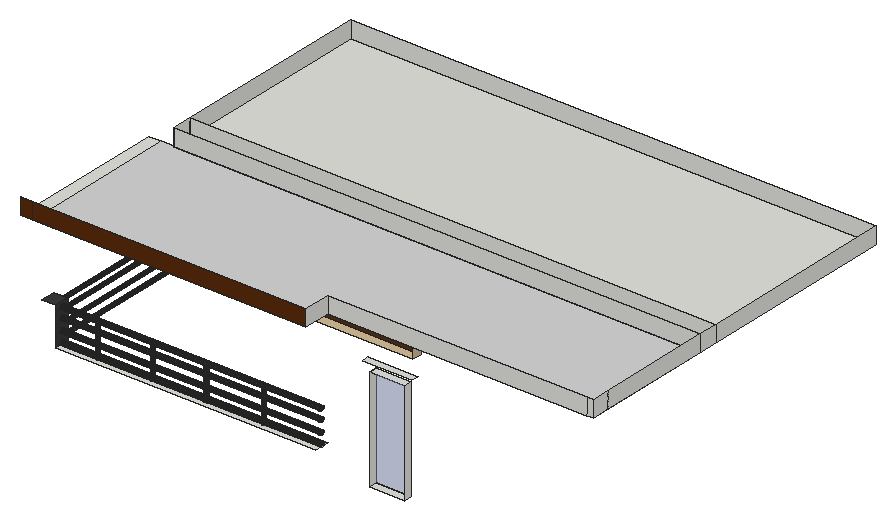
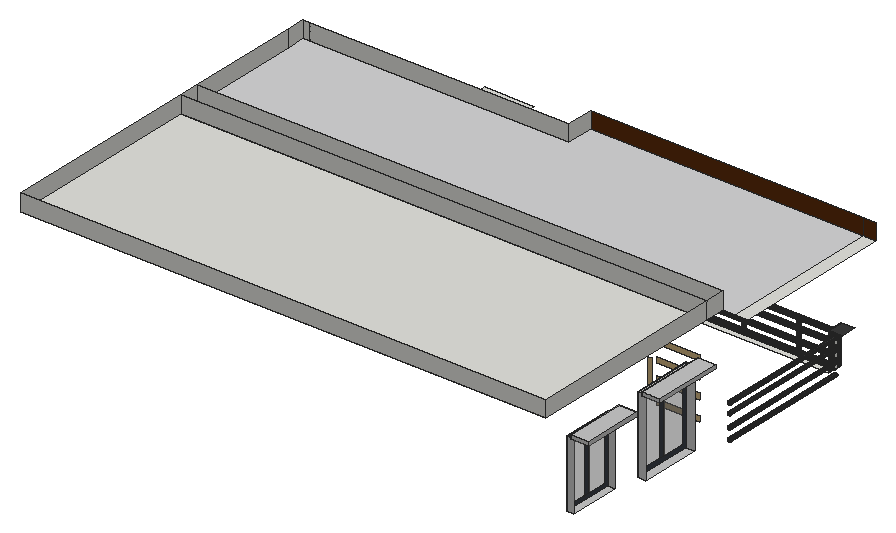
# SketchUp Ruby script. Lengths in inches.
U = 1.inch
M = Sketchup.active_model
def pt(a) = Geom::Point3d.new(a.map { |v| v * U })
def face(e, loops, mat)
  f = e.add_face(loops[0].map { |a| pt(a) })
  loops[1..].each { |l| e.add_face(l.map { |a| pt(a) }).erase! }
  f.material = f.back_material = mat if mat
  f
end
# faces: each face lists its corners as indices into pts; further lists are holes
def faces(e, pts, list, mat = nil) = list.each { |f| face(e, (f[0].is_a?(Array) ? f : [f]).map { |l| l.map { |i| pts[i] } }, mat) }
# xy, xz, yz: faces in a plane at the given z, y or x. An outline is a flat list of corners, or four numbers for a rectangle; further outlines are holes
def ring(l) = l.size == 4 ? [[l[0], l[1]], [l[2], l[1]], [l[2], l[3]], [l[0], l[3]]] : l.each_slice(2).to_a
def flat(e, list, mat, &to3) = list.each { |f| face(e, (f[0].is_a?(Array) ? f : [f]).map { |l| ring(l).map { |u, v| to3.(u, v) } }, mat) }
def xy(e, z, list, mat = nil) = flat(e, list, mat) { |x, y| [x, y, z] }
def xz(e, y, list, mat = nil) = flat(e, list, mat) { |x, z| [x, y, z] }
def yz(e, x, list, mat = nil) = flat(e, list, mat) { |y, z| [x, y, z] }
def lines(e, pts, list) = list.each { |a, b| e.add_line(pt(pts[a]), pt(pts[b])) }
# prism: a flat outline (further loops are holes) pulled along v
def prism(e, loops, v, mat = nil)
  f = face(e, loops, mat); d = Geom::Vector3d.new(v.map { |x| x * U })
  f.pushpull(f.normal.samedirection?(d) ? d.length : -d.length)
end
def box(e, o, s, mat = nil) = prism(e, [[o, [o[0] + s[0], o[1], o[2]], [o[0] + s[0], o[1] + s[1], o[2]], [o[0], o[1] + s[1], o[2]]]], [0, 0, s[2]], mat)
def at(x, y, z, deg = 0) = Geom::Transformation.translation(pt([x, y, z])) * Geom::Transformation.rotation(ORIGIN, Z_AXIS, deg.degrees)
def axes(o, x, y, z) = Geom::Transformation.new([*x, 0, *y, 0, *z, 0, *pt(o).to_a, 1])
def part(name) = M.definitions.add(name)
# library, detail: a bought-in or finely detailed component or shape, given as its bounding box
def library(name, o, s) = part(name).tap { |d| box(d.entities, o, s) }
def detail(e, o, s) = box(e.add_group.entities, o, s)
def put(e, d, t, mat = nil) = e.add_instance(d, t).tap { |i| i.material = mat if mat }
def group(e, t, mat = nil) = e.add_group.tap { |g| g.transformation = t; g.material = mat if mat }.entities
root = M.entities
M.materials.add("[0043_SaddleBrown]").color = [91, 44, 12]
M.materials.add("[Blinds Vertical Pattern]1").color = [212, 212, 214]
M.materials.add("[Color M02]").color = [198, 198, 198]
M.materials.add("[Color M07]").color = [58, 58, 58]
M.materials.add("[Formica Beige]").color = [211, 187, 149]
M.materials.add("[Formica Laminate Dark]").color = [59, 63, 71]
M.materials.add("[Translucent Glass Gray]").color = [128, 128, 128]
M.materials["[Translucent Glass Gray]"].alpha = 0.5
M.materials.add("[Translucent Glass Safety]").color = [204, 235, 244]
M.materials["[Translucent Glass Safety]"].alpha = 0.5
M.materials.add("[Translucent Glass Sky Reflection]").color = [126, 138, 183]
M.materials["[Translucent Glass Sky Reflection]"].alpha = 0.52
M.materials.add("[Wood Cherry Original]").color = [89, 50, 24]
M.materials.add("[Wood Floor Light]").color = [204, 176, 127]
xy(root,157.51,[[383.5,386.84,415.27,393.34]])
xy(root,157.625,[[[85.98,404.47,320.99,418.04],[216.94,409.26,216.54,409.31,216.17,409.45,215.85,409.67,215.61,409.95,215.46,410.28,215.4,410.64,215.46,410.99,215.61,411.33,215.85,411.61,216.17,411.83,216.54,411.97,216.94,412.01,217.34,411.97,217.71,411.83,218.03,411.61,218.28,411.33,218.43,410.99,218.48,410.64,218.43,410.28,218.28,409.95,218.03,409.67,217.71,409.45,217.34,409.31],[268.74,409.26,268.34,409.31,267.97,409.45,267.65,409.67,267.41,409.95,267.26,410.28,267.2,410.64,267.26,410.99,267.41,411.33,267.65,411.61,267.97,411.83,268.34,411.97,268.74,412.01,269.14,411.97,269.51,411.83,269.83,411.61,270.08,411.33,270.23,410.99,270.28,410.64,270.23,410.28,270.08,409.95,269.83,409.67,269.51,409.45,269.14,409.31],[168.5,409.26,168.1,409.31,167.73,409.45,167.41,409.67,167.17,409.95,167.02,410.28,166.96,410.64,167.02,410.99,167.17,411.33,167.41,411.61,167.73,411.83,168.1,411.97,168.5,412.01,168.9,411.97,169.27,411.83,169.59,411.61,169.84,411.33,169.99,410.99,170.04,410.64,169.99,410.28,169.84,409.95,169.59,409.67,169.27,409.45,168.9,409.31],[119.01,409.26,118.61,409.31,118.24,409.45,117.92,409.67,117.68,409.95,117.53,410.28,117.47,410.64,117.53,410.99,117.68,411.33,117.92,411.61,118.24,411.83,118.61,411.97,119.01,412.01,119.41,411.97,119.78,411.83,120.1,411.61,120.35,411.33,120.5,410.99,120.55,410.64,120.5,410.28,120.35,409.95,120.1,409.67,119.78,409.45,119.41,409.31]]])
xy(root,165.38,[[211.03,538.2,301.61,546.7]],"[Formica Beige]")
xy(root,172.06,[[73.92,584.76,81.73,639.13]],"[Color M02]")
xy(root,181.06,[[73.92,674.3125,80.55,720.75]],"[Color M02]")
xy(root,187.6875,[[80.02,508.58,80.47,508.63,80.89,508.79,81.25,509.04,81.53,509.36,81.71,509.74,81.77,510.14,81.71,510.55,81.53,510.92,81.25,511.25,80.89,511.49,80.47,511.65,80.02,511.7,79.56,511.65,79.14,511.49,78.78,511.25,78.5,510.92,78.33,510.55,78.27,510.14,78.33,509.74,78.5,509.36,78.78,509.04,79.14,508.79,79.56,508.63]])
xy(root,187.8125,[[80.02,443.08,80.47,443.13,80.89,443.29,81.25,443.54,81.53,443.86,81.71,444.24,81.77,444.64,81.71,445.05,81.53,445.42,81.25,445.75,80.89,445.99,80.47,446.15,80.02,446.2,79.56,446.15,79.14,445.99,78.78,445.75,78.5,445.42,78.33,445.05,78.27,444.64,78.33,444.24,78.5,443.86,78.78,443.54,79.14,443.29,79.56,443.13]])
xy(root,188.1875,[[80.02,477.83,80.47,477.88,80.89,478.04,81.25,478.29,81.53,478.61,81.71,478.99,81.77,479.39,81.71,479.8,81.53,480.17,81.25,480.5,80.89,480.74,80.47,480.9,80.02,480.95,79.56,480.9,79.14,480.74,78.78,480.5,78.5,480.17,78.33,479.8,78.27,479.39,78.33,478.99,78.5,478.61,78.78,478.29,79.14,478.04,79.56,477.88]])
xy(root,188.37,[[268.74,409.26,269.14,409.31,269.51,409.45,269.83,409.67,270.08,409.95,270.23,410.28,270.28,410.64,270.23,410.99,270.08,411.33,269.83,411.61,269.51,411.83,269.14,411.97,268.74,412.01,268.34,411.97,267.97,411.83,267.65,411.61,267.41,411.33,267.26,410.99,267.2,410.64,267.26,410.28,267.41,409.95,267.65,409.67,267.97,409.45,268.34,409.31]])
xy(root,188.375,[[168.5,409.26,168.9,409.31,169.27,409.45,169.59,409.67,169.84,409.95,169.99,410.28,170.04,410.64,169.99,410.99,169.84,411.33,169.59,411.61,169.27,411.83,168.9,411.97,168.5,412.01,168.1,411.97,167.73,411.83,167.41,411.61,167.17,411.33,167.02,410.99,166.96,410.64,167.02,410.28,167.17,409.95,167.41,409.67,167.73,409.45,168.1,409.31]])
xy(root,188.5,[[216.94,409.26,217.34,409.31,217.71,409.45,218.03,409.67,218.28,409.95,218.43,410.28,218.48,410.64,218.43,410.99,218.28,411.33,218.03,411.61,217.71,411.83,217.34,411.97,216.94,412.01,216.54,411.97,216.17,411.83,215.85,411.61,215.61,411.33,215.46,410.99,215.4,410.64,215.46,410.28,215.61,409.95,215.85,409.67,216.17,409.45,216.54,409.31]])
xy(root,188.85,[[119.01,409.26,119.41,409.31,119.78,409.45,120.1,409.67,120.35,409.95,120.5,410.28,120.55,410.64,120.5,410.99,120.35,411.33,120.1,411.61,119.78,411.83,119.41,411.97,119.01,412.01,118.61,411.97,118.24,411.83,117.92,411.61,117.68,411.33,117.53,410.99,117.47,410.64,117.53,410.28,117.68,409.95,117.92,409.67,118.24,409.45,118.61,409.31]])
xy(root,192.1875,[[73.92,404.47,85.98,418.04]],"[Color M07]")
xy(root,241.06,[[73.92,584.76,81.73,639.13]],"[Color M02]")
xy(root,241.56,[[73.92,674.3125,80.55,720.75]],"[Color M02]")
xy(root,242.21,[[57.67,580.82,73.92,643.76]],"[Color M02]")
xy(root,243.04,[[57.67,669.92,73.92,724.48]])
xy(root,246.02,[[57.67,580.82,73.92,643.76]],"[Color M02]")
xy(root,246.26,[[211.03,538.2,301.61,546.7]],"[Formica Beige]")
xy(root,246.66,[[57.67,669.92,73.92,724.48]],"[Color M02]")
xy(root,250.53,[[383.5,386.84,415.27,393.34]])
xy(root,257.08,[[376.94,386.84,421.82,393.34]])
xy(root,261.625,[[63.07,393.34,73.92,538.2],[85.98,538.2,560.26,556.28],[85.98,556.28,560.26,737.09]])
xy(root,261.625,[[73.92,393.34,73.92,538.2,560.26,538.2,560.26,418.04,320.99,418.04,320.99,393.34]],"[Blinds Vertical Pattern]1")
xz(root,393.34,[[63.07,261.625,73.92,276.4375],[73.92,261.625,320.99,276.4375]],"[0043_SaddleBrown]")
xz(root,393.34,[[383.5,157.51,415.27,250.53]],"[Translucent Glass Sky Reflection]")
xz(root,418.04,[[79.95,156.99,80.37,157.04,80.75,157.18,81.09,157.41,81.34,157.71,81.5,158.06,81.56,158.43,81.5,158.8,81.34,159.15,81.09,159.44,80.75,159.67,80.37,159.82,79.95,159.87,79.53,159.82,79.14,159.67,78.8125,159.44,78.55,159.15,78.39,158.8,78.34,158.43,78.39,158.06,78.55,157.71,78.8125,157.41,79.14,157.18,79.53,157.04],[79.95,166.99,80.37,167.04,80.75,167.18,81.09,167.41,81.34,167.71,81.5,168.06,81.56,168.43,81.5,168.8,81.34,169.15,81.09,169.44,80.75,169.67,80.37,169.82,79.95,169.87,79.53,169.82,79.14,169.67,78.8125,169.44,78.55,169.15,78.39,168.8,78.34,168.43,78.39,168.06,78.55,167.71,78.8125,167.41,79.14,167.18,79.53,167.04],[79.95,178.37,80.37,178.41,80.75,178.56,81.09,178.79,81.34,179.08,81.5,179.43,81.56,179.8,81.5,180.17,81.34,180.52,81.09,180.82,80.75,181.05,80.37,181.19,79.95,181.24,79.53,181.19,79.14,181.05,78.8125,180.82,78.55,180.52,78.39,180.17,78.34,179.8,78.39,179.43,78.55,179.08,78.8125,178.79,79.14,178.56,79.53,178.41],[79.95,186.93,80.37,186.98,80.75,187.12,81.09,187.35,81.34,187.65,81.5,187.99,81.56,188.37,81.5,188.74,81.34,189.08,81.09,189.38,80.75,189.61,80.37,189.75,79.95,189.8,79.53,189.75,79.14,189.61,78.8125,189.38,78.55,189.08,78.39,188.74,78.34,188.37,78.39,187.99,78.55,187.65,78.8125,187.35,79.14,187.12,79.53,186.98],[320.99,261.625,554.62,276.4375],
  [554.62,261.625,560.26,276.4375]])
xz(root,538.2,[[85.98,261.625,560.26,276.4375]])
xz(root,538.2,[[106.17,163.54,145.09,168.85],[149.97,173.81,153.54,199.88],[106.17,181.73,145.09,187.04],[106.17,197.6,145.09,202.92],[106.17,212.92,145.09,218.23]],"[Wood Floor Light]")
xz(root,546.7,[[215.15,169.06,233.62,242.58]],"[Translucent Glass Safety]")
xz(root,546.7,[[[211.03,165.38,301.61,246.26],[215.15,169.06,297.5,242.58]],[233.62,169.06,252.09,242.58],[252.09,169.06,257.69,242.58],[257.69,169.06,297.5,242.58]],"[Wood Cherry Original]")
xz(root,556.28,[[85.98,261.625,560.26,276.4375]])
xz(root,580.82,[[57.67,242.21,73.92,246.02]],"[Color M02]")
xz(root,584.76,[[73.92,172.06,81.73,241.06]],"[Color M02]")
xz(root,639.13,[[73.92,172.06,81.73,241.06]],"[Color M02]")
xz(root,643.76,[[57.67,242.21,73.92,246.02]],"[Color M02]")
xz(root,669.92,[[57.67,243.04,73.92,246.66]],"[Color M02]")
xz(root,674.3125,[[73.92,181.06,80.55,241.56]],"[Color M02]")
xz(root,720.75,[[73.92,181.06,80.55,241.56]],"[Color M02]")
xz(root,724.48,[[57.67,243.04,73.92,246.66]],"[Color M02]")
xz(root,737.09,[[85.98,261.625,560.26,276.4375]])
yz(root,57.67,[[580.82,242.21,643.76,246.02],[669.92,243.04,724.48,246.66]],"[Color M02]")
yz(root,73.92,[[580.82,242.21,643.76,246.02],[669.92,243.04,724.48,246.66]])
yz(root,80.55,[[[674.3125,181.06,720.75,241.56],[677.66,184.4,717.41,238.21]],[696.08,184.4,700.21,238.21]],"[Formica Laminate Dark]")
yz(root,80.55,[[677.66,184.4,696.08,238.21],[700.21,184.4,717.41,238.21]],"[Translucent Glass Gray]")
yz(root,81.73,[[[584.76,172.06,639.13,241.06],[588.66,175.95,635.24,237.16]],[610.13,175.95,614.62,237.16]],"[Formica Laminate Dark]")
yz(root,81.73,[[588.66,175.95,610.13,237.16],[614.62,175.95,635.24,237.16]],"[Translucent Glass Gray]")
yz(root,85.98,[[411.02,157.12,410.53,157.18,410.08,157.37,409.74,157.625,412.29,157.625,411.95,157.37,411.5,157.18],[409.74,157.625,409.69,157.67,409.39,158.06,409.2,158.51,409.14,158.99,409.2,159.48,409.39,159.93,409.69,160.32,410.08,160.62,410.53,160.8,411.02,160.87,411.5,160.8,411.95,160.62,412.34,160.32,412.64,159.93,412.83,159.48,412.89,158.99,412.83,158.51,412.64,158.06,412.34,157.67,412.29,157.625],[411.02,166.87,410.53,166.93,410.08,167.12,409.69,167.42,409.39,167.81,409.2,168.26,409.14,168.74,409.2,169.23,409.39,169.68,409.69,170.07,410.08,170.37,410.53,170.55,411.02,170.62,411.5,170.55,411.95,170.37,412.34,170.07,412.64,169.68,412.83,169.23,412.89,168.74,412.83,168.26,412.64,167.81,412.34,167.42,411.95,167.12,411.5,166.93],[411.02,177.37,410.53,177.43,410.08,177.62,409.69,177.92,409.39,178.31,409.2,178.76,409.14,179.24,409.2,179.73,409.39,180.18,409.69,180.57,410.08,180.87,410.53,181.05,411.02,181.12,411.5,181.05,411.95,180.87,412.34,180.57,412.64,180.18,412.83,179.73,412.89,179.24,412.83,178.76,412.64,178.31,412.34,177.92,411.95,177.62,411.5,177.43],[411.02,186.49,410.53,186.56,410.08,186.74,409.69,187.04,409.39,187.43,409.2,187.88,409.14,188.37,409.2,188.85,409.39,189.31,409.69,189.69,410.08,189.99,410.53,190.18,411.02,190.24,411.5,190.18,411.95,189.99,412.34,189.69,412.64,189.31,412.83,188.85,412.89,188.37,412.83,187.88,412.64,187.43,412.34,187.04,411.95,186.74,411.5,186.56],
  [538.2,261.625,556.28,276.4375],[556.28,261.625,737.09,276.4375]])
yz(root,85.98,[[[404.47,157.625,409.74,157.625,409.69,157.67,409.39,158.06,409.2,158.51,409.14,158.99,409.2,159.48,409.39,159.93,409.69,160.32,410.08,160.62,410.53,160.8,411.02,160.87,411.5,160.8,411.95,160.62,412.34,160.32,412.64,159.93,412.83,159.48,412.89,158.99,412.83,158.51,412.64,158.06,412.34,157.67,412.29,157.625,418.04,157.625,418.04,192.1875,404.47,192.1875],[411.02,166.87,410.53,166.93,410.08,167.12,409.69,167.42,409.39,167.81,409.2,168.26,409.14,168.74,409.2,169.23,409.39,169.68,409.69,170.07,410.08,170.37,410.53,170.55,411.02,170.62,411.5,170.55,411.95,170.37,412.34,170.07,412.64,169.68,412.83,169.23,412.89,168.74,412.83,168.26,412.64,167.81,412.34,167.42,411.95,167.12,411.5,166.93],[411.02,177.37,410.53,177.43,410.08,177.62,409.69,177.92,409.39,178.31,409.2,178.76,409.14,179.24,409.2,179.73,409.39,180.18,409.69,180.57,410.08,180.87,410.53,181.05,411.02,181.12,411.5,181.05,411.95,180.87,412.34,180.57,412.64,180.18,412.83,179.73,412.89,179.24,412.83,178.76,412.64,178.31,412.34,177.92,411.95,177.62,411.5,177.43],[411.02,186.49,410.53,186.56,410.08,186.74,409.69,187.04,409.39,187.43,409.2,187.88,409.14,188.37,409.2,188.85,409.39,189.31,409.69,189.69,410.08,189.99,410.53,190.18,411.02,190.24,411.5,190.18,411.95,189.99,412.34,189.69,412.64,189.31,412.83,188.85,412.89,188.37,412.83,187.88,412.64,187.43,412.34,187.04,411.95,186.74,411.5,186.56]]],"[Color M07]")
yz(root,211.03,[[538.2,165.38,546.7,246.26]],"[Formica Beige]")
yz(root,301.61,[[538.2,165.38,546.7,246.26]],"[Formica Beige]")
yz(root,320.99,[[411.02,157.12,411.5,157.18,411.95,157.37,412.29,157.625,409.74,157.625,410.08,157.37,410.53,157.18],[393.34,261.625,418.04,276.4375]])
yz(root,383.5,[[386.84,157.51,393.34,250.53]])
yz(root,415.27,[[386.84,157.51,393.34,250.53]])
yz(root,560.26,[[418.04,261.625,434.85,276.4375],[434.85,261.625,538.2,276.4375],[538.2,261.625,556.28,276.4375],[556.28,261.625,737.09,276.4375]])
p = [[79.53,418.04,157.04],[79.14,418.04,157.18],[79.14,538.2,157.18],[79.53,538.2,157.04],[79.95,418.04,156.99],[79.95,538.2,156.99],
  [80.37,418.04,157.04],[80.37,538.2,157.04],[80.75,418.04,157.18],[80.75,538.2,157.18],[85.98,410.53,157.18],[85.98,411.02,157.12],
  [320.99,411.02,157.12],[320.99,410.53,157.18],[85.98,411.5,157.18],[320.99,411.5,157.18],[85.98,410.08,157.37],[320.99,410.08,157.37],
  [85.98,411.95,157.37],[320.99,411.95,157.37],[78.8125,418.04,157.41],[78.8125,538.2,157.41],[81.09,418.04,157.41],[81.09,538.2,157.41],
  [85.98,409.74,157.625],[320.99,409.74,157.625],[320.99,409.69,157.67],[85.98,409.69,157.67],[85.98,412.29,157.625],[85.98,412.34,157.67],
  [320.99,412.34,157.67],[320.99,412.29,157.625],[78.55,418.04,157.71],[78.55,538.2,157.71],[81.34,418.04,157.71],[81.34,538.2,157.71],
  [118.24,409.45,188.85],[118.24,409.45,157.625],[118.61,409.31,157.625],[118.61,409.31,188.85],[119.01,409.26,157.625],[119.01,409.26,188.85],
  [119.41,409.31,157.625],[119.41,409.31,188.85],[119.78,409.45,157.625],[119.78,409.45,188.85],[167.73,409.45,188.375],[167.73,409.45,157.625],
  [168.1,409.31,157.625],[168.1,409.31,188.375],[168.5,409.26,157.625],[168.5,409.26,188.375],[168.9,409.31,157.625],[168.9,409.31,188.375],
  [169.27,409.45,157.625],[169.27,409.45,188.375],[216.17,409.45,188.5],[216.17,409.45,157.625],[216.54,409.31,157.625],[216.54,409.31,188.5],
  [216.94,409.26,157.625],[216.94,409.26,188.5],[217.34,409.31,157.625],[217.34,409.31,188.5],[217.71,409.45,157.625],[217.71,409.45,188.5],
  [267.97,409.45,188.37],[267.97,409.45,157.625],[268.34,409.31,157.625],[268.34,409.31,188.37],[268.74,409.26,157.625],[268.74,409.26,188.37],
  [269.14,409.31,157.625],[269.14,409.31,188.37],[269.51,409.45,157.625],[269.51,409.45,188.37],[117.92,409.67,188.85],[117.92,409.67,157.625],
  [120.1,409.67,157.625],[120.1,409.67,188.85],[167.41,409.67,188.375],[167.41,409.67,157.625],[169.59,409.67,157.625],[169.59,409.67,188.375],
  [215.85,409.67,188.5],[215.85,409.67,157.625],[218.03,409.67,157.625],[218.03,409.67,188.5],[267.65,409.67,188.37],[267.65,409.67,157.625],
  [269.83,409.67,157.625],[269.83,409.67,188.37],[117.68,409.95,188.85],[117.68,409.95,157.625],[120.35,409.95,157.625],[120.35,409.95,188.85],
  [167.17,409.95,188.375],[167.17,409.95,157.625],[169.84,409.95,157.625],[169.84,409.95,188.375],[215.61,409.95,188.5],[215.61,409.95,157.625],
  [218.28,409.95,157.625],[218.28,409.95,188.5],[267.41,409.95,188.37],[267.41,409.95,157.625],[270.08,409.95,157.625],[270.08,409.95,188.37],
  [117.53,410.28,188.85],[117.53,410.28,157.625],[120.5,410.28,157.625],[120.5,410.28,188.85],[167.02,410.28,188.375],[167.02,410.28,157.625],
  [169.99,410.28,157.625],[169.99,410.28,188.375],[215.46,410.28,188.5],[215.46,410.28,157.625],[218.43,410.28,157.625],[218.43,410.28,188.5],
  [267.26,410.28,188.37],[267.26,410.28,157.625],[270.23,410.28,157.625],[270.23,410.28,188.37],[117.47,410.64,188.85],[117.47,410.64,157.625],
  [120.55,410.64,157.625],[120.55,410.64,188.85],[166.96,410.64,188.375],[166.96,410.64,157.625],[170.04,410.64,157.625],[170.04,410.64,188.375],
  [215.4,410.64,188.5],[215.4,410.64,157.625],[218.48,410.64,157.625],[218.48,410.64,188.5],[267.2,410.64,188.37],[267.2,410.64,157.625],
  [270.28,410.64,157.625],[270.28,410.64,188.37],[117.53,410.99,188.85],[117.53,410.99,157.625],[120.5,410.99,157.625],[120.5,410.99,188.85],
  [167.02,410.99,188.375],[167.02,410.99,157.625],[169.99,410.99,157.625],[169.99,410.99,188.375],[215.46,410.99,188.5],[215.46,410.99,157.625],
  [218.43,410.99,157.625],[218.43,410.99,188.5],[267.26,410.99,188.37],[267.26,410.99,157.625],[270.23,410.99,157.625],[270.23,410.99,188.37],
  [117.68,411.33,188.85],[117.68,411.33,157.625],[120.35,411.33,157.625],[120.35,411.33,188.85],[167.17,411.33,188.375],[167.17,411.33,157.625],
  [169.84,411.33,157.625],[169.84,411.33,188.375],[215.61,411.33,188.5],[215.61,411.33,157.625],[218.28,411.33,157.625],[218.28,411.33,188.5],
  [267.41,411.33,188.37],[267.41,411.33,157.625],[270.08,411.33,157.625],[270.08,411.33,188.37],[117.92,411.61,188.85],[117.92,411.61,157.625],
  [120.1,411.61,157.625],[120.1,411.61,188.85],[167.41,411.61,188.375],[167.41,411.61,157.625],[169.59,411.61,157.625],[169.59,411.61,188.375],
  [215.85,411.61,188.5],[215.85,411.61,157.625],[218.03,411.61,157.625],[218.03,411.61,188.5],[267.65,411.61,188.37],[267.65,411.61,157.625],
  [269.83,411.61,157.625],[269.83,411.61,188.37],[118.24,411.83,188.85],[118.24,411.83,157.625],[119.78,411.83,157.625],[119.78,411.83,188.85],
  [167.73,411.83,188.375],[167.73,411.83,157.625],[169.27,411.83,157.625],[169.27,411.83,188.375],[216.17,411.83,188.5],[216.17,411.83,157.625],
  [217.71,411.83,157.625],[217.71,411.83,188.5],[267.97,411.83,188.37],[267.97,411.83,157.625],[269.51,411.83,157.625],[269.51,411.83,188.37],
  [118.61,411.97,188.85],[118.61,411.97,157.625],[119.41,411.97,157.625],[119.41,411.97,188.85],[168.1,411.97,188.375],[168.1,411.97,157.625],
  [168.9,411.97,157.625],[168.9,411.97,188.375],[216.54,411.97,188.5],[216.54,411.97,157.625],[217.34,411.97,157.625],[217.34,411.97,188.5],
  [268.34,411.97,188.37],[268.34,411.97,157.625],[269.14,411.97,157.625],[269.14,411.97,188.37],[119.01,412.01,188.85],[119.01,412.01,157.625],
  [168.5,412.01,188.375],[168.5,412.01,157.625],[216.94,412.01,188.5],[216.94,412.01,157.625],[268.74,412.01,188.37],[268.74,412.01,157.625],
  [85.98,409.39,158.06],[320.99,409.39,158.06],[85.98,412.64,158.06],[320.99,412.64,158.06],[78.39,418.04,158.06],[78.39,538.2,158.06],
  [81.5,418.04,158.06],[81.5,538.2,158.06],[85.98,409.2,158.51],[320.99,409.2,158.51],[85.98,412.83,158.51],[320.99,412.83,158.51],
  [78.34,418.04,158.43],[78.34,538.2,158.43],[81.56,418.04,158.43],[81.56,538.2,158.43],[78.39,418.04,158.8],[78.39,538.2,158.8],
  [81.5,418.04,158.8],[81.5,538.2,158.8],[85.98,409.14,158.99],[320.99,409.14,158.99],[85.98,412.89,158.99],[320.99,412.89,158.99],
  [78.55,418.04,159.15],[78.55,538.2,159.15],[81.34,418.04,159.15],[81.34,538.2,159.15],[85.98,409.2,159.48],[320.99,409.2,159.48],
  [85.98,412.83,159.48],[320.99,412.83,159.48],[78.8125,418.04,159.44],[78.8125,538.2,159.44],[81.09,418.04,159.44],[81.09,538.2,159.44],
  [79.14,418.04,159.67],[79.14,538.2,159.67],[80.75,418.04,159.67],[80.75,538.2,159.67],[85.98,409.39,159.93],[320.99,409.39,159.93],
  [85.98,412.64,159.93],[320.99,412.64,159.93],[79.53,418.04,159.82],[79.53,538.2,159.82],[80.37,418.04,159.82],[80.37,538.2,159.82],
  [79.95,418.04,159.87],[79.95,538.2,159.87],[85.98,409.69,160.32],[320.99,409.69,160.32],[85.98,412.34,160.32],[320.99,412.34,160.32],
  [85.98,410.08,160.62],[320.99,410.08,160.62],[85.98,411.95,160.62],[320.99,411.95,160.62],[85.98,410.53,160.8],[320.99,410.53,160.8],
  [85.98,411.5,160.8],[320.99,411.5,160.8],[85.98,411.02,160.87],[320.99,411.02,160.87],[85.98,410.08,167.12],[85.98,410.53,166.93],
  [320.99,410.53,166.93],[320.99,410.08,167.12],[85.98,411.02,166.87],[320.99,411.02,166.87],[85.98,411.5,166.93],[320.99,411.5,166.93],
  [85.98,411.95,167.12],[320.99,411.95,167.12],[79.53,418.04,167.04],[79.14,418.04,167.18],[79.14,538.2,167.18],[79.53,538.2,167.04],
  [79.95,418.04,166.99],[79.95,538.2,166.99],[80.37,418.04,167.04],[80.37,538.2,167.04],[80.75,418.04,167.18],[80.75,538.2,167.18],
  [85.98,409.69,167.42],[320.99,409.69,167.42],[85.98,412.34,167.42],[320.99,412.34,167.42],[78.8125,418.04,167.41],[78.8125,538.2,167.41],
  [81.09,418.04,167.41],[81.09,538.2,167.41],[85.98,409.39,167.81],[320.99,409.39,167.81],[85.98,412.64,167.81],[320.99,412.64,167.81],
  [78.55,418.04,167.71],[78.55,538.2,167.71],[81.34,418.04,167.71],[81.34,538.2,167.71],[78.39,418.04,168.06],[78.39,538.2,168.06],
  [81.5,418.04,168.06],[81.5,538.2,168.06],[85.98,409.2,168.26],[320.99,409.2,168.26],[85.98,412.83,168.26],[320.99,412.83,168.26],
  [78.34,418.04,168.43],[78.34,538.2,168.43],[81.56,418.04,168.43],[81.56,538.2,168.43],[85.98,409.14,168.74],[320.99,409.14,168.74],
  [85.98,412.89,168.74],[320.99,412.89,168.74],[78.39,418.04,168.8],[78.39,538.2,168.8],[81.5,418.04,168.8],[81.5,538.2,168.8],
  [85.98,409.2,169.23],[320.99,409.2,169.23],[85.98,412.83,169.23],[320.99,412.83,169.23],[78.55,418.04,169.15],[78.55,538.2,169.15],
  [81.34,418.04,169.15],[81.34,538.2,169.15],[78.8125,418.04,169.44],[78.8125,538.2,169.44],[81.09,418.04,169.44],[81.09,538.2,169.44],
  [85.98,409.39,169.68],[320.99,409.39,169.68],[85.98,412.64,169.68],[320.99,412.64,169.68],[79.14,418.04,169.67],[79.14,538.2,169.67],
  [80.75,418.04,169.67],[80.75,538.2,169.67],[85.98,409.69,170.07],[320.99,409.69,170.07],[85.98,412.34,170.07],[320.99,412.34,170.07],
  [79.53,418.04,169.82],[79.53,538.2,169.82],[80.37,418.04,169.82],[80.37,538.2,169.82],[79.95,418.04,169.87],[79.95,538.2,169.87],
  [85.98,410.08,170.37],[320.99,410.08,170.37],[85.98,411.95,170.37],[320.99,411.95,170.37],[85.98,410.53,170.55],[320.99,410.53,170.55],
  [85.98,411.5,170.55],[320.99,411.5,170.55],[85.98,411.02,170.62],[320.99,411.02,170.62],[85.98,410.08,177.62],[85.98,410.53,177.43],
  [320.99,410.53,177.43],[320.99,410.08,177.62],[85.98,411.02,177.37],[320.99,411.02,177.37],[85.98,411.5,177.43],[320.99,411.5,177.43],
  [85.98,411.95,177.62],[320.99,411.95,177.62],[85.98,409.69,177.92],[320.99,409.69,177.92],[85.98,412.34,177.92],[320.99,412.34,177.92],
  [85.98,409.39,178.31],[320.99,409.39,178.31],[85.98,412.64,178.31],[320.99,412.64,178.31],[85.98,409.2,178.76],[320.99,409.2,178.76],
  [85.98,412.83,178.76],[320.99,412.83,178.76],[79.53,418.04,178.41],[79.14,418.04,178.56],[79.14,538.2,178.56],[79.53,538.2,178.41],
  [79.95,418.04,178.37],[79.95,538.2,178.37],[80.37,418.04,178.41],[80.37,538.2,178.41],[80.75,418.04,178.56],[80.75,538.2,178.56],
  [78.8125,418.04,178.79],[78.8125,538.2,178.79],[81.09,418.04,178.79],[81.09,538.2,178.79],[85.98,409.14,179.24],[320.99,409.14,179.24],
  [85.98,412.89,179.24],[320.99,412.89,179.24],[78.55,418.04,179.08],[78.55,538.2,179.08],[81.34,418.04,179.08],[81.34,538.2,179.08],
  [78.39,418.04,179.43],[78.39,538.2,179.43],[81.5,418.04,179.43],[81.5,538.2,179.43],[85.98,409.2,179.73],[320.99,409.2,179.73],
  [85.98,412.83,179.73],[320.99,412.83,179.73],[78.34,418.04,179.8],[78.34,538.2,179.8],[81.56,418.04,179.8],[81.56,538.2,179.8],
  [85.98,409.39,180.18],[320.99,409.39,180.18],[85.98,412.64,180.18],[320.99,412.64,180.18],[78.39,418.04,180.17],[78.39,538.2,180.17],
  [81.5,418.04,180.17],[81.5,538.2,180.17],[85.98,409.69,180.57],[320.99,409.69,180.57],[85.98,412.34,180.57],[320.99,412.34,180.57],
  [78.55,418.04,180.52],[78.55,538.2,180.52],[81.34,418.04,180.52],[81.34,538.2,180.52],[78.8125,418.04,180.82],[78.8125,538.2,180.82],
  [81.09,418.04,180.82],[81.09,538.2,180.82],[85.98,410.08,180.87],[320.99,410.08,180.87],[85.98,411.95,180.87],[320.99,411.95,180.87],
  [79.14,418.04,181.05],[79.14,538.2,181.05],[80.75,418.04,181.05],[80.75,538.2,181.05],[85.98,410.53,181.05],[320.99,410.53,181.05],
  [85.98,411.5,181.05],[320.99,411.5,181.05],[79.53,418.04,181.19],[79.53,538.2,181.19],[80.37,418.04,181.19],[80.37,538.2,181.19],
  [85.98,411.02,181.12],[320.99,411.02,181.12],[79.95,418.04,181.24],[79.95,538.2,181.24],[85.98,410.53,186.56],[85.98,411.02,186.49],
  [320.99,411.02,186.49],[320.99,410.53,186.56],[85.98,411.5,186.56],[320.99,411.5,186.56],[85.98,410.08,186.74],[320.99,410.08,186.74],
  [85.98,411.95,186.74],[320.99,411.95,186.74],[85.98,409.69,187.04],[320.99,409.69,187.04],[85.98,412.34,187.04],[320.99,412.34,187.04],
  [79.95,418.04,186.93],[79.53,418.04,186.98],[79.53,538.2,186.98],[79.95,538.2,186.93],[80.37,418.04,186.98],[80.37,538.2,186.98],
  [85.98,409.39,187.43],[320.99,409.39,187.43],[85.98,412.64,187.43],[320.99,412.64,187.43],[79.14,418.04,187.12],[79.14,538.2,187.12],
  [80.75,418.04,187.12],[80.75,538.2,187.12],[78.8125,418.04,187.35],[78.8125,538.2,187.35],[81.09,418.04,187.35],[81.09,538.2,187.35],
  [78.55,418.04,187.65],[78.55,538.2,187.65],[81.34,418.04,187.65],[81.34,538.2,187.65],[85.98,409.2,187.88],[320.99,409.2,187.88],
  [85.98,412.83,187.88],[320.99,412.83,187.88],[78.39,418.04,187.99],[78.39,538.2,187.99],[81.5,418.04,187.99],[81.5,538.2,187.99],
  [85.98,409.14,188.37],[320.99,409.14,188.37],[85.98,412.89,188.37],[320.99,412.89,188.37],[78.34,418.04,188.37],[78.34,538.2,188.37],
  [81.56,418.04,188.37],[81.56,538.2,188.37],[85.98,409.2,188.85],[320.99,409.2,188.85],[85.98,412.83,188.85],[320.99,412.83,188.85],
  [78.39,418.04,188.74],[78.39,538.2,188.74],[81.5,418.04,188.74],[81.5,538.2,188.74],[78.55,418.04,189.08],[78.55,538.2,189.08],
  [81.34,418.04,189.08],[81.34,538.2,189.08],[85.98,409.39,189.31],[320.99,409.39,189.31],[85.98,412.64,189.31],[320.99,412.64,189.31],
  [78.8125,418.04,189.38],[78.8125,538.2,189.38],[81.09,418.04,189.38],[81.09,538.2,189.38],[85.98,409.69,189.69],[320.99,409.69,189.69],
  [85.98,412.34,189.69],[320.99,412.34,189.69],[79.14,418.04,189.61],[79.14,538.2,189.61],[80.75,418.04,189.61],[80.75,538.2,189.61],
  [79.53,418.04,189.75],[79.53,538.2,189.75],[80.37,418.04,189.75],[80.37,538.2,189.75],[85.98,410.08,189.99],[320.99,410.08,189.99],
  [85.98,411.95,189.99],[320.99,411.95,189.99],[79.95,418.04,189.8],[79.95,538.2,189.8],[85.98,410.53,190.18],[320.99,410.53,190.18],
  [85.98,411.5,190.18],[320.99,411.5,190.18],[85.98,411.02,190.24],[320.99,411.02,190.24]]
faces(root,p,[[0,1,2,3],[4,0,3,5],[6,4,5,7],[8,6,7,9],[10,11,12,13],[11,14,15,12],[16,10,13,17],[14,18,19,15],
  [1,20,21,2],[22,8,9,23],[24,16,17,25,26,27],[28,29,30,31,19,18],[20,32,33,21],[34,22,23,35],[36,37,38,39],[39,38,40,41],
  [41,40,42,43],[43,42,44,45],[46,47,48,49],[49,48,50,51],[51,50,52,53],[53,52,54,55],[56,57,58,59],[59,58,60,61],
  [61,60,62,63],[63,62,64,65],[66,67,68,69],[69,68,70,71],[71,70,72,73],[73,72,74,75],[76,77,37,36],[45,44,78,79],
  [80,81,47,46],[55,54,82,83],[84,85,57,56],[65,64,86,87],[88,89,67,66],[75,74,90,91],[92,93,77,76],[79,78,94,95],
  [96,97,81,80],[83,82,98,99],[100,101,85,84],[87,86,102,103],[104,105,89,88],[91,90,106,107],[108,109,93,92],[95,94,110,111],
  [112,113,97,96],[99,98,114,115],[116,117,101,100],[103,102,118,119],[120,121,105,104],[107,106,122,123],[124,125,109,108],[111,110,126,127],
  [128,129,113,112],[115,114,130,131],[132,133,117,116],[119,118,134,135],[136,137,121,120],[123,122,138,139],[140,141,125,124],[127,126,142,143],
  [144,145,129,128],[131,130,146,147],[148,149,133,132],[135,134,150,151],[152,153,137,136],[139,138,154,155],[156,157,141,140],[143,142,158,159],
  [160,161,145,144],[147,146,162,163],[164,165,149,148],[151,150,166,167],[168,169,153,152],[155,154,170,171],[172,173,157,156],[159,158,174,175],
  [176,177,161,160],[163,162,178,179],[180,181,165,164],[167,166,182,183],[184,185,169,168],[171,170,186,187],[188,189,173,172],[175,174,190,191],
  [192,193,177,176],[179,178,194,195],[196,197,181,180],[183,182,198,199],[200,201,185,184],[187,186,202,203],[204,205,189,188],[191,190,206,207],
  [208,209,193,192],[195,194,210,211],[212,213,197,196],[199,198,214,215],[216,217,201,200],[203,202,218,219],[220,221,205,204],[207,206,221,220],
  [222,223,209,208],[211,210,223,222],[224,225,213,212],[215,214,225,224],[226,227,217,216],[219,218,227,226],[228,27,26,229],[29,230,231,30],
  [32,232,233,33],[234,34,35,235],[236,228,229,237],[230,238,239,231],[232,240,241,233],[242,234,235,243],[240,244,245,241],[246,242,243,247],
  [248,236,237,249],[238,250,251,239],[244,252,253,245],[254,246,247,255],[256,248,249,257],[250,258,259,251],[252,260,261,253],[262,254,255,263],
  [260,264,265,261],[266,262,263,267],[268,256,257,269],[258,270,271,259],[264,272,273,265],[274,266,267,275],[272,276,277,273],[276,274,275,277],
  [278,268,269,279],[270,280,281,271],[282,278,279,283],[280,284,285,281],[286,282,283,287],[284,288,289,285],[290,286,287,291],[288,290,291,289],
  [292,293,294,295],[293,296,297,294],[296,298,299,297],[298,300,301,299],[302,303,304,305],[306,302,305,307],[308,306,307,309],[310,308,309,311],
  [312,292,295,313],[300,314,315,301],[303,316,317,304],[318,310,311,319],[320,312,313,321],[314,322,323,315],[316,324,325,317],[326,318,319,327],
  [324,328,329,325],[330,326,327,331],[332,320,321,333],[322,334,335,323],[328,336,337,329],[338,330,331,339],[340,332,333,341],[334,342,343,335],
  [336,344,345,337],[346,338,339,347],[348,340,341,349],[342,350,351,343],[344,352,353,345],[354,346,347,355],[352,356,357,353],[358,354,355,359],
  [360,348,349,361],[350,362,363,351],[356,364,365,357],[366,358,359,367],[368,360,361,369],[362,370,371,363],[364,372,373,365],[374,366,367,375],
  [372,376,377,373],[376,374,375,377],[378,368,369,379],[370,380,381,371],[382,378,379,383],[380,384,385,381],[386,382,383,387],[384,386,387,385],
  [388,389,390,391],[389,392,393,390],[392,394,395,393],[394,396,397,395],[398,388,391,399],[396,400,401,397],[402,398,399,403],[400,404,405,401],
  [406,402,403,407],[404,408,409,405],[410,411,412,413],[414,410,413,415],[416,414,415,417],[418,416,417,419],[411,420,421,412],[422,418,419,423],
  [424,406,407,425],[408,426,427,409],[420,428,429,421],[430,422,423,431],[428,432,433,429],[434,430,431,435],[436,424,425,437],[426,438,439,427],
  [432,440,441,433],[442,434,435,443],[444,436,437,445],[438,446,447,439],[440,448,449,441],[450,442,443,451],[452,444,445,453],[446,454,455,447],
  [448,456,457,449],[458,450,451,459],[456,460,461,457],[462,458,459,463],[464,452,453,465],[454,466,467,455],[460,468,469,461],[470,462,463,471],
  [472,464,465,473],[466,474,475,467],[468,476,477,469],[478,470,471,479],[480,472,473,481],[474,480,481,475],[476,482,483,477],[482,478,479,483],
  [484,485,486,487],[485,488,489,486],[490,484,487,491],[488,492,493,489],[494,490,491,495],[492,496,497,493],[498,499,500,501],[502,498,501,503],
  [504,494,495,505],[496,506,507,497],[499,508,509,500],[510,502,503,511],[508,512,513,509],[514,510,511,515],[512,516,517,513],[518,514,515,519],
  [520,504,505,521],[506,522,523,507],[516,524,525,517],[526,518,519,527],[528,520,521,529],[522,530,531,523],[524,532,533,525],[534,526,527,535],
  [536,528,529,537],[530,538,539,531],[532,540,541,533],[542,534,535,543],[540,544,545,541],[546,542,543,547],[548,536,537,549],[538,550,551,539],
  [544,552,553,545],[554,546,547,555],[556,548,549,557],[550,558,559,551],[552,560,561,553],[562,554,555,563],[560,564,565,561],[566,562,563,567],
  [568,556,557,569],[558,570,571,559],[564,572,573,565],[572,566,567,573],[574,568,569,575],[570,576,577,571],[578,574,575,579],[576,578,579,577]],"[Color M07]")
